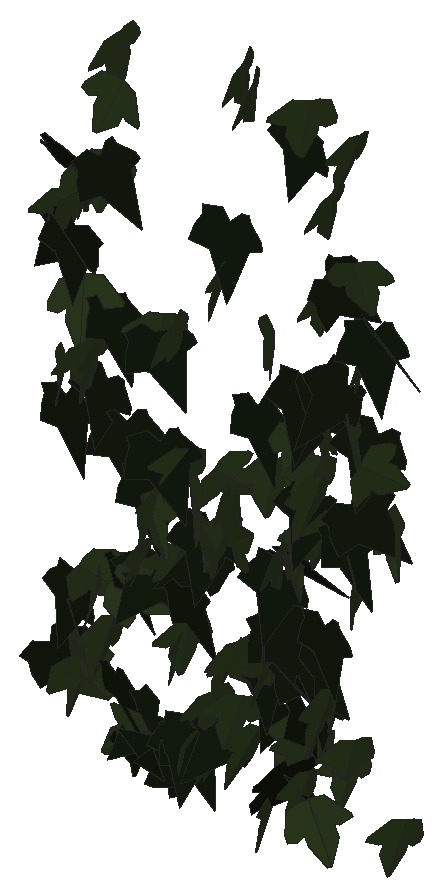
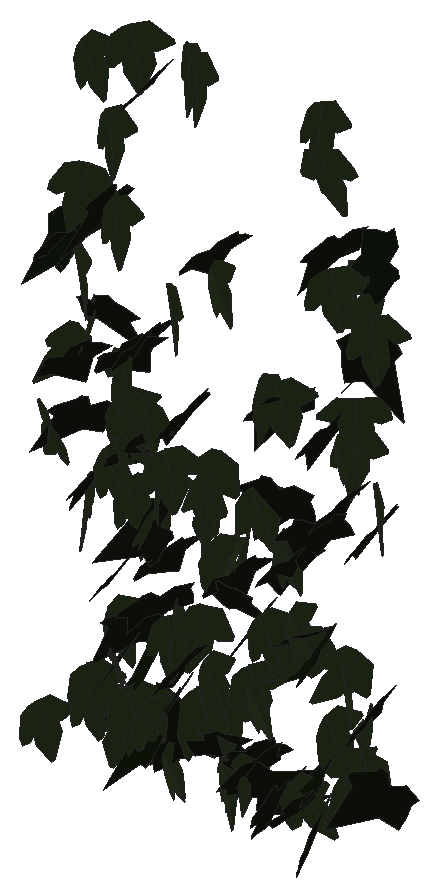
# SketchUp Ruby script. Lengths in inches.
U = 1.inch
M = Sketchup.active_model
def pt(a) = Geom::Point3d.new(a.map { |v| v * U })
def face(e, loops, mat)
  f = e.add_face(loops[0].map { |a| pt(a) })
  loops[1..].each { |l| e.add_face(l.map { |a| pt(a) }).erase! }
  f.material = f.back_material = mat if mat
  f
end
# faces: each face lists its corners as indices into pts; further lists are holes
def faces(e, pts, list, mat = nil) = list.each { |f| face(e, (f[0].is_a?(Array) ? f : [f]).map { |l| l.map { |i| pts[i] } }, mat) }
# xy, xz, yz: faces in a plane at the given z, y or x. An outline is a flat list of corners, or four numbers for a rectangle; further outlines are holes
def ring(l) = l.size == 4 ? [[l[0], l[1]], [l[2], l[1]], [l[2], l[3]], [l[0], l[3]]] : l.each_slice(2).to_a
def flat(e, list, mat, &to3) = list.each { |f| face(e, (f[0].is_a?(Array) ? f : [f]).map { |l| ring(l).map { |u, v| to3.(u, v) } }, mat) }
def xy(e, z, list, mat = nil) = flat(e, list, mat) { |x, y| [x, y, z] }
def xz(e, y, list, mat = nil) = flat(e, list, mat) { |x, z| [x, y, z] }
def yz(e, x, list, mat = nil) = flat(e, list, mat) { |y, z| [x, y, z] }
def lines(e, pts, list) = list.each { |a, b| e.add_line(pt(pts[a]), pt(pts[b])) }
# prism: a flat outline (further loops are holes) pulled along v
def prism(e, loops, v, mat = nil)
  f = face(e, loops, mat); d = Geom::Vector3d.new(v.map { |x| x * U })
  f.pushpull(f.normal.samedirection?(d) ? d.length : -d.length)
end
def box(e, o, s, mat = nil) = prism(e, [[o, [o[0] + s[0], o[1], o[2]], [o[0] + s[0], o[1] + s[1], o[2]], [o[0], o[1] + s[1], o[2]]]], [0, 0, s[2]], mat)
def at(x, y, z, deg = 0) = Geom::Transformation.translation(pt([x, y, z])) * Geom::Transformation.rotation(ORIGIN, Z_AXIS, deg.degrees)
def axes(o, x, y, z) = Geom::Transformation.new([*x, 0, *y, 0, *z, 0, *pt(o).to_a, 1])
def part(name) = M.definitions.add(name)
# library, detail: a bought-in or finely detailed component or shape, given as its bounding box
def library(name, o, s) = part(name).tap { |d| box(d.entities, o, s) }
def detail(e, o, s) = box(e.add_group.entities, o, s)
def put(e, d, t, mat = nil) = e.add_instance(d, t).tap { |i| i.material = mat if mat }
def group(e, t, mat = nil) = e.add_group.tap { |g| g.transformation = t; g.material = mat if mat }.entities
root = M.entities
M.materials.add("efeu1").color = [18, 25, 13]
M.materials.add("efeu2").color = [43, 57, 29]
c1 = part("ivyleaf_10")
p = [[0,0.5,-0.03],[-0.0625,2.02,-0.43],[-0.19,2.01,-0.46],[-0.54,1.05,-0.29],[-0.52,0.625,-0.18],[-0.83,0.76,-0.28],
  [-1.16,0.64,-0.33],[-1.15,0.33,-0.24],[-0.77,-0.39,0.02],[-0.3,-0.51,0.16],[0.04,-0.48,0.23],[-0.02,2.01,-0.4375],
  [-0.06,2.01,-0.43],[0.04,-0.49,0.23],[0.67,-0.49,0.14],[1.38,0.36,-0.2],[1.375,0.51,-0.24],[0.81,0.65,-0.19],
  [0.62,0.59,-0.15],[0.6,1.09,-0.28],[0.5,1.23,-0.31]]
faces(c1.entities,p,[[0,1,2,3,4,5,6,7,8,9,10],[11,12,0,13,14,15,16,17,18,19,20]],"efeu2")
c2 = part("ivyleaf_9")
p = [[1.54,2.16,1.25],[1.36,2.04,1.19],[-0.21,0.99,0.68],[-0.71,1.11,0.82],[-0.85,0.86,0.67],[-0.8,0.17,0.21],
  [-0.9,-0.01,0.1],[-0.67,-0.16,-0.02],[-0.08,-0.08,-0.05],[-0.03,-0.6,-0.4],[0.65,-0.88,-0.66],[0.83,-0.6,-0.49],
  [1.29,-0.42,-0.43],[1.8125,-0.07,-0.26],[1.21,0.44,0.15]]
faces(c2.entities,p,[[0,1,2,3,4,5,6,7,8,9,10,11,12,13,14]],"efeu1")
put(root,c1,axes([546.2,128.18,259.55],[0.61192,-0.80627,-0.41024],[-0.13377,0.40919,-1.00374],[0.89469,0.61263,0.13051]))
put(root,c2,axes([545.57,128.43,246.6875],[-0.00928,-0.23007,-1.06512],[0.36964,1.00134,-0.21951],[1.02507,-0.36316,0.06952]))
put(root,c1,axes([546.3,128.39,267.17],[-0.51603,-0.96649,0.0334],[-0.01193,-0.0315,-1.09562],[0.967,-0.51615,0.00431]))
put(root,c2,axes([546.93,128.01,266.18],[0.38492,0.23675,-1.07574],[-0.89278,-0.60038,-0.45158],[-0.64516,0.97207,-0.01691]))
put(root,c2,axes([546.52,128.64,249.48],[-0.02237,-0.91012,0.53359],[-0.02809,-0.53301,-0.91031],[1.05464,-0.0335,-0.01292]))
put(root,c2,axes([546.34,128.31,258.07],[0.34407,-1.06382,-0.00474],[-0.00139,0.00453,-1.11808],[1.06383,0.34407,0.00007]))
put(root,c2,axes([546.56,128.375,265.49],[0.0872,-1.02644,0.33344],[0.12969,-0.32214,-1.02556],[1.07142,0.12253,0.097]))
put(root,c2,axes([546.4,127.41,269.83],[1.06067,-0.29857,0.25163],[0.24243,-0.06743,-1.10189],[0.30609,1.08802,0.00076]))
put(root,c1,axes([547.18,127.24,268.04],[-0.0161,-0.263,-1.09291],[0.2004,1.07484,-0.2616],[1.1061,-0.19856,0.03148]))
put(root,c1,axes([546.67,128.21,248.2],[0.10603,-0.24599,1.06458],[0.98076,-0.45001,-0.20167],[0.4816,0.9706,0.1763]))
put(root,c1,axes([547.2,128.26,263.34],[0.91449,0.73038,-0.01547],[-0.01203,-0.00973,-1.17036],[-0.73045,0.91457,-0.00009]))
put(root,c1,axes([547.375,128.19,246.71],[0.21173,-0.93259,0.56746],[0.25398,-0.52009,-0.94951],[1.06171,0.3104,0.11397]))
put(root,c1,axes([547.36,127.67,246.72],[-0.67476,-0.71201,-0.63835],[0.45877,0.44445,-0.98068],[0.83903,-0.81563,0.02286]))
put(root,c1,axes([547.9375,128.91,269.06],[-0.68312,-0.83444,0.20316],[0.03779,-0.28855,-1.05808],[0.85799,-0.65166,0.20836]))
put(root,c1,axes([547.93,127.66,268.85],[0.47058,-0.88521,-0.483],[-0.09372,0.4923,-0.99357],[1.00404,0.46084,0.13363]))
put(root,c1,axes([547.93,127.51,261.2],[-0.32602,-1.04852,-0.2068],[0.0382,0.20464,-1.09778],[1.06804,-0.32738,-0.02386]))
put(root,c2,axes([547.66,129.17,258.93],[-0.0791,-1.0106,0.33071],[0.04958,-0.33477,-1.01114],[1.06217,-0.05963,0.07183]))
put(root,c1,axes([548.14,127.94,261],[0.35776,-0.99235,0.27961],[0.09809,-0.26186,-1.05486],[1.02631,0.37095,0.00335]))
put(root,c1,axes([548.45,127.52,250.62],[0.39264,-0.81638,-0.65059],[-0.30369,0.5757,-0.90568],[0.99875,0.496,-0.01962]))
put(root,c1,axes([547.92,127.72,251.18],[-0.47149,-0.54655,-0.78965],[0.58759,0.53162,-0.7188],[0.7596,-0.75048,0.06589]))
put(root,c1,axes([548.35,128.44,248.4],[0.02393,-1.10375,0.38166],[0.09584,-0.37859,-1.1009],[1.16393,0.05387,0.08281]))
put(root,c2,axes([548.07,129.07,262.42],[0.26023,-1.02512,-0.25312],[-0.07183,0.2429,-1.05759],[1.05346,0.26979,-0.00958]))
put(root,c2,axes([548.86,129.6,242.89],[-0.1823,-0.08431,1.02203],[-0.15312,-1.02417,-0.1118],[1.014,-0.16981,0.16686]))
put(root,c2,axes([548.76,127.57,270.05],[0.27574,-0.86201,-0.65588],[-0.06367,0.66273,-0.89778],[1.08129,0.25885,0.1144]))
put(root,c2,axes([548.99,128.8,257.6],[-0.2672,-0.92808,-0.50235],[0.14797,0.48014,-0.96574],[1.04489,-0.30532,0.0083]))
put(root,c1,axes([549.5,127.48,273.41],[1.06147,-0.00633,-0.42592],[-0.41653,0.22396,-1.0414],[0.08916,1.12159,0.20554]))
put(root,c2,axes([548.71,128.54,246.26],[0.5542,-0.86163,0.22518],[0.11681,-0.1926,-1.02445],[0.88287,0.56634,-0.0058]))
put(root,c1,axes([549.43,127.74,275.58],[-0.16093,-1.08433,-0.26183],[0.08223,0.25229,-1.09536],[1.11246,-0.17551,0.04309]))
put(root,c1,axes([550.35,127.98,244.53],[-0.63086,-0.1592,0.89678],[-0.84685,-0.29902,-0.64882],[0.33525,-1.05489,0.04858]))
put(root,c2,axes([549.15,128.29,251.56],[0.64938,-0.80947,-0.00179],[-0.00104,0.00145,-1.03776],[0.80947,0.64938,0.0001]))
put(root,c2,axes([549.9375,129.38,244.48],[-0.47114,-0.69278,0.63141],[-0.15949,-0.63713,-0.81806],[0.92368,-0.46338,0.18081]))
put(root,c1,axes([550.17,128.42,252.57],[0.27751,-0.93345,0.37983],[0.0903,-0.36935,-0.97367],[1.00371,0.29131,-0.01742]))
put(root,c1,axes([549.92,127.46,251.16],[0.22752,0.55169,1.03329],[0.40948,0.94872,-0.59671],[-1.09744,0.46837,-0.00843]))
put(root,c2,axes([550.18,128.86,255.57],[0.01979,-1.06474,-0.17642],[0.01626,0.17673,-1.06475],[1.07914,0.01686,0.01928]))
put(root,c1,axes([550.82,128.76,262.82],[-0.58054,-0.8867,0.28565],[-0.06802,-0.29533,-1.055],[0.92909,-0.57567,0.10125]))
put(root,c2,axes([550.63,128.66,251.62],[-0.63278,-0.75503,0.33523],[0.03135,-0.44392,-0.94065],[0.82551,-0.5619,0.29269]))
put(root,c1,axes([551.16,129.1875,252.34],[-0.16179,-0.97806,0.34417],[-0.01494,-0.3461,-0.99056],[1.03674,-0.15762,0.03943]))
put(root,c1,axes([551.09,128.1,255.4],[0.28882,-0.95997,0.405],[0.11829,-0.38734,-1.00247],[1.03516,0.3121,0.00156]))
put(root,c2,axes([550.84,128.44,262.43],[0.05059,-0.93908,-0.57946],[0.04279,0.5813,-0.93833],[1.10264,0.02052,0.063]))
put(root,c1,axes([550.96,127.875,255.02],[-0.81857,0.17952,-0.63499],[0.49843,-0.49483,-0.78243],[-0.43244,-0.91017,0.30014]))
put(root,c1,axes([551.54,128.52,262.82],[0.07679,-0.99229,-0.44675],[0.0796,0.45178,-0.98979],[1.08531,0.03708,0.1042]))
put(root,c2,axes([551.63,128.88,243.28],[-0.26053,-0.15666,1.01123],[-0.38686,-0.95097,-0.24699],[0.94735,-0.43142,0.17724]))
put(root,c1,axes([551.68,129.15,248.99],[0.45181,-0.92911,0.29151],[0.09086,-0.27974,-1.0324],[0.96952,0.45919,-0.0391]))
put(root,c2,axes([552.4,127.92,243.71],[-0.0302,0.01725,1.01443],[-1.01355,0.04513,-0.03094],[-0.04563,-1.01388,0.01588]))
put(root,c2,axes([551.41,127.95,257.92],[-0.46501,-0.58652,-0.85049],[0.54507,0.65302,-0.74836],[0.87763,-0.71633,0.01415]))
put(root,c1,axes([552.18,128.72,249.47],[-0.39396,-0.96695,0.11113],[-0.01812,-0.11258,-1.04381],[0.97314,-0.39355,0.02555]))
put(root,c1,axes([552.25,128.41,257.38],[-0.3352,-0.97831,0.34484],[-0.07161,-0.33971,-1.03336],[1.03483,-0.3404,0.04019]))
put(root,c1,axes([552.47,128.69,255.91],[-0.38407,0.87166,-0.47073],[0.14349,-0.4506,-0.95146],[-0.9802,-0.40751,0.04517]))
put(root,c2,axes([553.4,129.07,253.13],[-1.00334,0.05538,0.27568],[-0.27811,-0.04482,-1.0032],[-0.04146,-1.03956,0.05794]))
put(root,c1,axes([553.02,127.6,244.76],[-0.00213,0.70633,0.73753],[-0.48292,0.64916,-0.62308],[-0.8998,-0.35008,0.33267]))
put(root,c2,axes([552.47,128.3125,245.29],[0.259,-1.03557,-0.41472],[-0.06271,0.41156,-1.06684],[1.11376,0.26399,0.03637]))
put(root,c2,axes([552.46,128.09,251.6],[0.58906,-0.86857,-0.22769],[-0.09983,0.20727,-1.04896],[0.89235,0.59655,0.03295]))
put(root,c2,axes([552.96,127.98,245.51],[-0.42066,-0.93913,-0.16507],[0.05248,0.15734,-1.02891],[0.95208,-0.42361,-0.01622]))
put(root,c2,axes([552.97,129.06,254.08],[-0.26077,-1.0379,0.06941],[-0.00202,-0.07105,-1.07005],[1.04022,-0.26033,0.01532]))
put(root,c1,axes([553.57,128.62,244.73],[0.3666,-1.07233,-0.23436],[-0.0506,0.23031,-1.13297],[1.09648,0.36916,0.02607]))
put(root,c1,axes([553.84,128.98,254.61],[-0.10631,-0.96679,0.45959],[0.04955,-0.4658,-0.96839],[1.06932,-0.07453,0.09057]))
put(root,c1,axes([553.89,128.09,247.3],[-0.29235,-0.9761,-0.13873],[0.02003,0.13879,-1.01873],[0.9857,-0.29232,-0.02044]))
put(root,c1,axes([553.57,128.42,253.91],[-0.57085,0.30448,0.89081],[0.58976,-0.69636,0.61595],[0.73378,0.79656,0.19796]))
put(root,c1,axes([554.17,128.85,249.12],[0.15964,-1.00517,0.26184],[0.03185,-0.26005,-1.01772],[1.03822,0.16253,-0.00904]))
put(root,c2,axes([554.43,128.75,245.84],[-0.85647,-0.54311,0.17545],[-0.11054,-0.15257,-1.01183],[0.55994,-0.86085,0.06863]))
put(root,c1,axes([554.26,128.36,266.66],[0.3844,-0.99544,0.22732],[0.06835,-0.21726,-1.06698],[1.01877,0.39017,-0.01418]))
put(root,c1,axes([554.42,128.56,256.6875],[0.21652,-0.95794,-0.47403],[0.0522,0.49256,-0.97155],[1.06754,0.1702,0.14365]))
put(root,c2,axes([554.08,128.93,268.38],[-0.11894,-1.08675,-0.01996],[0.06594,0.01283,-1.09136],[1.08493,-0.11992,0.06414]))
put(root,c1,axes([554.59,127.83,257.88],[-0.40988,-0.64076,-0.76736],[0.41678,0.64432,-0.76064],[0.90869,-0.58455,0.00274]))
put(root,c1,axes([555.07,128.3,247.31],[-0.47232,-0.87369,0.2882],[-0.10444,-0.27095,-0.99255],[0.91405,-0.48242,0.03552]))
put(root,c1,axes([555.2,128.32,276.02],[0.199,-1.02755,-0.40769],[-0.00501,0.4134,-1.04439],[1.10546,0.18685,0.06866]))
put(root,c1,axes([555.66,128.26,246.05],[0.10168,-0.89329,0.61369],[0.088,-0.60755,-0.89893],[1.08021,0.13357,0.01546]))
put(root,c1,axes([555.69,127.38,250.36],[-0.4708,-0.85884,-0.41169],[0.16686,0.37776,-0.97887],[0.93768,-0.49843,-0.03252]))
put(root,c1,axes([555.19,127.81,254.86],[-0.67486,0.17521,0.84981],[0.83133,-0.1778,0.69684],[0.24853,1.07051,-0.02335]))
put(root,c2,axes([555.45,129.36,249.05],[0.13703,-1.05273,0.13672],[0.01338,-0.13613,-1.06161],[1.06149,0.13761,-0.00426]))
put(root,c2,axes([555.47,128.97,260.5],[0.27086,-1.05188,-0.0887],[-0.01264,0.08833,-1.08615],[1.05554,0.27098,0.00975]))
put(root,c1,axes([556.18,129.0625,258.03],[-0.57816,-0.91228,0.16133],[0.03586,-0.21206,-1.07065],[0.92574,-0.56154,0.14223]))
put(root,c1,axes([556.26,127.52,275.79],[0.23128,-0.97472,-0.53381],[-0.08187,0.52882,-1.00109],[1.1083,0.24247,0.03744]))
put(root,c2,axes([555.79,129.67,247.06],[0.00277,-0.77898,0.71508],[0.04607,-0.71431,-0.77832],[1.05642,0.0332,0.03206]))
put(root,c1,axes([556.39,128.69,250.23],[-0.32362,-1.00449,-0.06189],[-0.00111,0.06537,-1.05512],[1.00639,-0.32294,-0.02106]))
put(root,c1,axes([557.04,127.21,250.02],[0.09545,-0.52779,-0.96309],[-0.21909,0.93814,-0.53583],[1.07615,0.2378,-0.02367]))
put(root,c1,axes([556.97,127.81,264.73],[0.71078,-0.66199,-0.52453],[-0.21544,0.52077,-0.94919],[0.81667,0.71354,0.20613]))
put(root,c2,axes([556.67,128.93,253.52],[-0.24041,-1.04013,0.19968],[-0.00886,-0.20277,-1.06694],[1.05909,-0.23781,0.0364]))
put(root,c1,axes([556.8125,128.15,243.71],[0.43069,-0.85807,0.41051],[0.19185,-0.36301,-0.96006],[0.93167,0.47142,0.00792]))
put(root,c1,axes([557,129.44,246.33],[-0.12719,-0.77001,0.67294],[0.25344,-0.68071,-0.73099],[0.99072,0.07528,0.27339]))
put(root,c2,axes([556.9375,128.69,251.46],[0.086,-1.05613,-0.5701],[0.11474,0.57618,-1.05009],[1.19468,0.02069,0.14189]))
put(root,c1,axes([557.37,128.66,254.97],[-0.34129,1.00124,-0.06655],[0.02263,-0.06259,-1.05781],[-1.00319,-0.34204,-0.00122]))
put(root,c1,axes([557.66,127.54,255.38],[0.26347,-0.99616,-0.40747],[-0.03775,0.41069,-1.02844],[1.07562,0.25842,0.06371]))
put(root,c1,axes([557.44,128.77,259.93],[1.05338,-0.18903,0.03298],[0.05132,0.10023,-1.06478],[0.18489,1.04912,0.10766]))
put(root,c2,axes([557.41,127.02,244.84],[-0.00531,0.96764,-0.6836],[-0.09298,0.68116,0.96491],[1.1811,0.05798,0.07289]))
put(root,c2,axes([557.09,128.58,254.62],[1.03529,-0.06916,0.21352],[0.21933,0.09786,-1.03175],[0.04764,1.05254,0.10996]))
put(root,c2,axes([557.45,128.48,244.95],[0.95051,-0.23897,-0.31139],[-0.24799,0.26675,-0.96171],[0.30425,0.96399,0.18892]))
put(root,c1,axes([558.08,129.08,246.46],[-0.38621,-1.05676,0.39393],[-0.09494,-0.38444,-1.12439],[1.12379,-0.39565,0.04039]))
put(root,c1,axes([558.08,129.05,255.97],[-0.17773,-0.95896,0.42217],[0.1137,-0.44332,-0.95914],[1.04159,-0.11524,0.17674]))
put(root,c2,axes([558.05,128.86,247.23],[-0.28074,-0.40803,0.92483],[0.09591,-0.96626,-0.39719],[1.00628,-0.02174,0.29587]))
put(root,c2,axes([557.85,128.7,250.14],[0.09355,-0.6302,-0.83409],[0.22059,0.83046,-0.60273],[1.02186,-0.12158,0.20647]))
put(root,c2,axes([558.125,128.55,262.5],[-0.06099,-1.09203,0.20003],[-0.0105,-0.19976,-1.09373],[1.11015,-0.06188,0.00065]))
put(root,c1,axes([558.47,128.125,245.1],[0.04679,-1.00017,0.32262],[0.09766,-0.3174,-0.99816],[1.04637,0.07435,0.07873]))
put(root,c2,axes([558.18,128.53,273.87],[-0.10126,-0.97599,0.52165],[0.06886,-0.52837,-0.9752],[1.10451,-0.05654,0.10862]))
put(root,c2,axes([558.16,129.57,248.7],[0.2015,-0.94978,0.45185],[0.0875,-0.44334,-0.97091],[1.04814,0.2196,-0.00582]))
put(root,c1,axes([558.85,128.42,259.33],[-0.2864,-0.94984,0.42976],[-0.02129,-0.44026,-0.98724],[1.04233,-0.26998,0.09792]))
put(root,c1,axes([558.99,127.75,275.78],[-0.64492,-0.93034,0.15816],[-0.04365,-0.16194,-1.13064],[0.94268,-0.64398,0.05584]))
put(root,c2,axes([558.73,128.85,262.12],[-0.46111,-0.97307,0.1304],[-0.043,-0.12391,-1.07671],[0.98083,-0.4629,0.0141]))
put(root,c2,axes([558.63,128.63,257.61],[-0.27741,-1.00563,0.23315],[-0.03898,-0.23105,-1.04294],[1.03157,-0.27917,0.02329]))
put(root,c1,axes([558.95,128.48,261.26],[-0.91723,0.56518,0.07249],[-0.09704,-0.01957,-1.07526],[-0.56149,-0.91988,0.06741]))
put(root,c1,axes([559,128.09,258.44],[0.13422,-1.0736,0.58604],[0.20564,-0.56136,-1.07548],[1.20572,0.21525,0.11819]))
put(root,c1,axes([559.28,128.86,256.89],[-0.03461,-1.04937,0.32883],[-0.02416,-0.32818,-1.04986],[1.09942,-0.04025,-0.01272]))
put(root,c1,axes([559.15,128.86,248.3],[0.77789,-0.67667,0.3183],[0.2133,-0.23943,-1.03029],[0.71673,0.80567,-0.03884]))
put(root,c2,axes([559.06,128.72,251.95],[0.23838,-1.02478,0.17504],[0.05771,-0.16626,-1.05198],[1.03802,0.24458,0.01829]))
put(root,c1,axes([559.63,127.99,267.7],[0.04273,-1.1123,-0.13027],[0.02134,0.13115,-1.11281],[1.1197,0.03994,0.02618]))
put(root,c1,axes([559.67,128,249.23],[0.19886,-1.10467,0.40504],[0.12675,-0.38828,-1.12119],[1.16974,0.22987,0.05263]))
put(root,c1,axes([559.8,128.08,271.84],[0.0761,-1.0816,-0.29426],[-0.03185,0.29273,-1.08422],[1.12046,0.08178,-0.01084]))
put(root,c1,axes([559.34,127.51,244.25],[0.82529,0.61188,0.42349],[0.33674,0.25685,-1.02737],[-0.66358,0.89133,0.00534]))
put(root,c1,axes([560.02,129.17,246.16],[-0.29283,-0.95672,0.26524],[0.09605,-0.30254,-0.98522],[0.98815,-0.2541,0.17437]))
put(root,c2,axes([560.32,128.33,263.48],[-1.05444,-0.26332,-0.06963],[0.0639,0.03147,-1.08672],[0.26477,-1.05627,-0.01501]))
put(root,c1,axes([560.23,128.94,246.85],[-0.40448,-0.93336,0.14182],[-0.02916,-0.14186,-1.01681],[0.94362,-0.40447,0.02937]))
put(root,c2,axes([559.91,127.91,268.35],[0.46943,-0.40472,-0.9178],[-0.37805,0.86722,-0.57578],[0.9291,0.55736,0.22944]))
put(root,c2,axes([559.82,128.92,256.375],[0.39129,-0.98507,-0.26716],[-0.03406,0.27336,-1.05781],[1.02009,0.38699,0.06716]))
put(root,c1,axes([560.79,128.25,254.82],[0.57086,-0.66517,-0.85461],[-0.16905,0.8995,-0.81303],[1.06969,0.49713,0.32759]))
put(root,c1,axes([560.93,128.21,274.66],[0.09776,-1.07825,0.26087],[-0.01027,-0.26275,-1.08217],[1.10931,0.09259,-0.03301]))
put(root,c1,axes([561.04,128.55,265.2],[0.54062,-0.95786,-0.16865],[-0.00591,0.18972,-1.09644],[0.97258,0.5336,0.08709]))
put(root,c1,axes([561.0625,128.27,268.98],[-0.98058,-0.49484,-0.17897],[0.15002,0.0999,-1.09815],[0.50437,-0.99176,-0.02132]))
put(root,c1,axes([561.2,127.66,262.25],[-0.54117,0.92083,-0.21138],[0.08677,-0.19413,-1.06783],[-0.94078,-0.54759,0.02311]))
put(root,c2,axes([561.25,129.21,261.17],[-0.40465,-1.00898,0.01705],[0.0068,-0.02109,-1.087],[1.0091,-0.40446,0.01416]))
put(root,c2,axes([561.02,128.07,258.42],[0.25783,-0.61874,-0.88905],[0.16954,0.92568,-0.59506],[1.06981,0.00242,0.30856]))
put(root,c2,axes([561.74,128.44,266.26],[-0.03814,-1.08994,-0.24088],[0.0012,0.24098,-1.09058],[1.11624,-0.0375,-0.00706]))
put(root,c2,axes([561.625,128.5,266.47],[1.02373,-0.3629,-0.18858],[-0.1726,0.07747,-1.08604],[0.37077,1.03807,0.01512]))
put(root,c1,axes([562.27,127.47,260.86],[-0.18545,-0.69008,-0.87003],[0.48732,0.74203,-0.69243],[0.99784,-0.49065,0.17647]))
put(root,c1,axes([561.92,129.17,257.5],[0.78769,-0.25929,0.7659],[0.72045,-0.26042,-0.82911],[0.36713,1.06736,-0.01623]))
put(root,c1,axes([562.84,128.85,244.18],[-0.3375,-0.95975,0.26741],[-0.0184,-0.27629,-1.01482],[0.99613,-0.33028,0.07186]))
